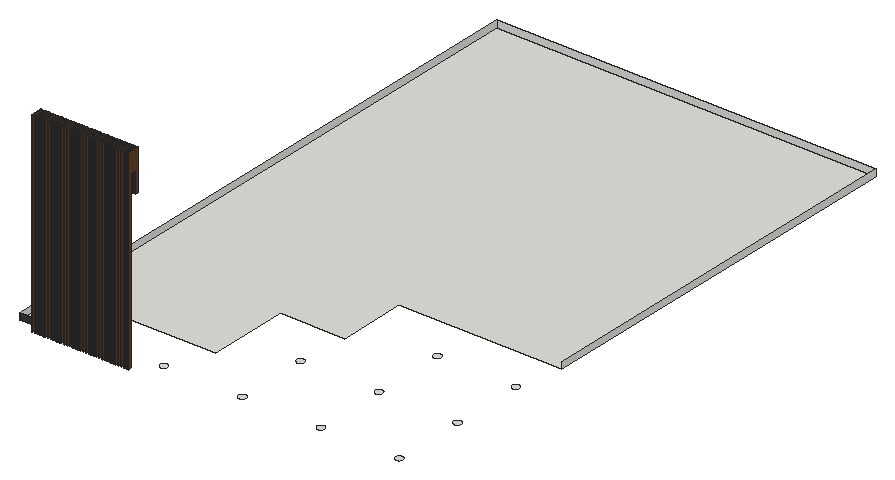
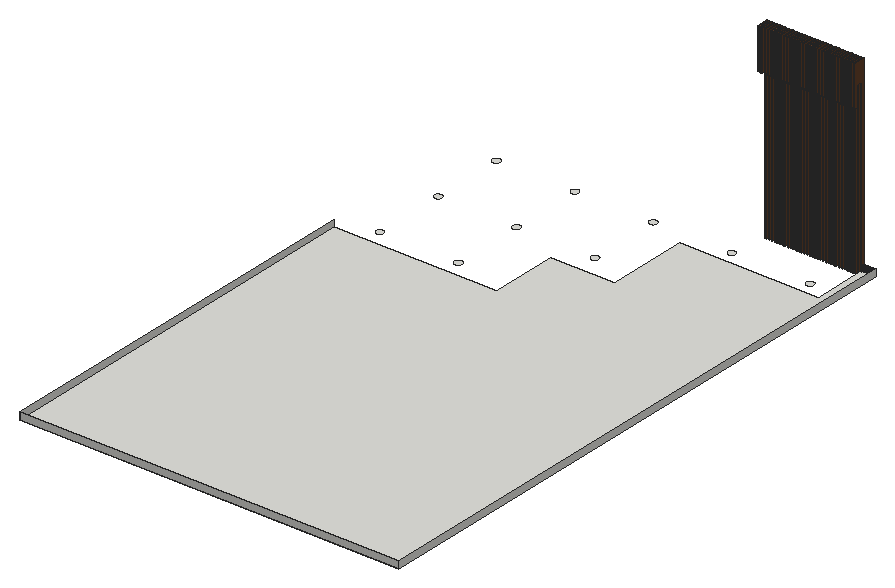
# SketchUp Ruby script. Lengths in inches.
U = 1.inch
M = Sketchup.active_model
def pt(a) = Geom::Point3d.new(a.map { |v| v * U })
def face(e, loops, mat)
  f = e.add_face(loops[0].map { |a| pt(a) })
  loops[1..].each { |l| e.add_face(l.map { |a| pt(a) }).erase! }
  f.material = f.back_material = mat if mat
  f
end
# faces: each face lists its corners as indices into pts; further lists are holes
def faces(e, pts, list, mat = nil) = list.each { |f| face(e, (f[0].is_a?(Array) ? f : [f]).map { |l| l.map { |i| pts[i] } }, mat) }
# xy, xz, yz: faces in a plane at the given z, y or x. An outline is a flat list of corners, or four numbers for a rectangle; further outlines are holes
def ring(l) = l.size == 4 ? [[l[0], l[1]], [l[2], l[1]], [l[2], l[3]], [l[0], l[3]]] : l.each_slice(2).to_a
def flat(e, list, mat, &to3) = list.each { |f| face(e, (f[0].is_a?(Array) ? f : [f]).map { |l| ring(l).map { |u, v| to3.(u, v) } }, mat) }
def xy(e, z, list, mat = nil) = flat(e, list, mat) { |x, y| [x, y, z] }
def xz(e, y, list, mat = nil) = flat(e, list, mat) { |x, z| [x, y, z] }
def yz(e, x, list, mat = nil) = flat(e, list, mat) { |y, z| [x, y, z] }
def lines(e, pts, list) = list.each { |a, b| e.add_line(pt(pts[a]), pt(pts[b])) }
# prism: a flat outline (further loops are holes) pulled along v
def prism(e, loops, v, mat = nil)
  f = face(e, loops, mat); d = Geom::Vector3d.new(v.map { |x| x * U })
  f.pushpull(f.normal.samedirection?(d) ? d.length : -d.length)
end
def box(e, o, s, mat = nil) = prism(e, [[o, [o[0] + s[0], o[1], o[2]], [o[0] + s[0], o[1] + s[1], o[2]], [o[0], o[1] + s[1], o[2]]]], [0, 0, s[2]], mat)
def at(x, y, z, deg = 0) = Geom::Transformation.translation(pt([x, y, z])) * Geom::Transformation.rotation(ORIGIN, Z_AXIS, deg.degrees)
def axes(o, x, y, z) = Geom::Transformation.new([*x, 0, *y, 0, *z, 0, *pt(o).to_a, 1])
def part(name) = M.definitions.add(name)
# library, detail: a bought-in or finely detailed component or shape, given as its bounding box
def library(name, o, s) = part(name).tap { |d| box(d.entities, o, s) }
def detail(e, o, s) = box(e.add_group.entities, o, s)
def put(e, d, t, mat = nil) = e.add_instance(d, t).tap { |i| i.material = mat if mat }
def group(e, t, mat = nil) = e.add_group.tap { |g| g.transformation = t; g.material = mat if mat }.entities
root = M.entities
M.materials.add("1432 AP 8245 TAR ROAD").color = [57, 57, 60]
M.materials.add("[Wood Veneer 01]").color = [99, 65, 42]
c1 = part("2")
prism(c1.entities,[[[0,1.5,0],[0,-0.5,0],[0,-0.5,172],[0,9.5,172],[0,9.5,136],[0,7.5,136],[0,7.5,154],[0,1.5,154]]],[1.5,0,0])
xy(root,111,[[50.84,185,50.76,185.01,50.6875,185.02,50.61,185.03,50.45,185.05,50.375,185.07,50.3,185.08,50.22,185.1,50.15,185.125,50.07,185.15,50,185.17,49.92,185.2,49.71,185.29,49.64,185.33,49.57,185.36,49.43,185.44,49.37,185.48,49.3,185.53,49.24,185.57,49.17,185.62,48.93,185.82,48.88,185.88,48.82,185.93,48.62,186.17,48.57,186.24,48.53,186.3,48.48,186.37,48.44,186.43,48.36,186.57,48.33,186.64,48.29,186.71,48.2,186.92,48.17,187,48.15,187.07,48.125,187.15,48.1,187.22,48.08,187.3,48.07,187.375,48.05,187.45,48.03,187.61,48.02,187.6875,48.01,187.76,48,187.84,48,188.16,48.01,188.24,48.02,188.3125,48.03,188.39,48.05,188.55,48.07,188.625,48.08,188.7,48.1,188.78,48.125,188.85,48.15,188.93,48.17,189,48.2,189.08,48.29,189.29,48.33,189.36,48.36,189.43,48.44,189.57,48.48,189.63,48.53,189.7,48.57,189.76,48.62,189.83,48.82,190.07,48.88,190.12,48.93,190.18,49.17,190.38,49.24,190.43,49.3,190.47,49.37,190.52,49.43,190.56,49.57,190.64,49.64,190.67,49.71,190.71,49.92,190.8,50,190.83,50.07,190.85,50.15,190.875,50.22,190.9,50.3,190.92,50.375,190.93,50.45,190.95,50.61,190.97,50.6875,190.98,50.76,190.99,50.84,191,51.16,191,51.24,190.99,51.3125,190.98,51.39,190.97,51.55,190.95,51.625,190.93,51.7,190.92,51.78,190.9,51.85,190.875,51.93,190.85,52,190.83,52.08,190.8,52.29,190.71,52.36,190.67,52.43,190.64,52.57,190.56,52.63,190.52,52.7,190.47,52.76,190.43,52.83,190.38,53.07,190.18,53.12,190.12,53.18,190.07,53.38,189.83,53.43,189.76,53.47,189.7,53.52,189.63,53.56,189.57,53.64,189.43,53.67,189.36,53.71,189.29,53.8,189.08,53.83,189,53.85,188.93,53.875,188.85,53.9,188.78,53.92,188.7,53.93,188.625,53.95,188.55,53.97,188.39,53.98,188.3125,53.99,188.24,54,188.16,54,187.84,53.99,187.76,53.98,187.6875,53.97,187.61,53.95,187.45,53.93,187.375,53.92,187.3,53.9,187.22,53.875,187.15,53.85,187.07,53.83,187,53.8,186.92,53.71,186.71,53.67,186.64,53.64,186.57,53.56,186.43,53.52,186.37,53.47,186.3,53.43,186.24,53.38,186.17,53.18,185.93,53.12,185.88,53.07,185.82,52.83,185.62,52.76,185.57,52.7,185.53,52.63,185.48,52.57,185.44,52.43,185.36,52.36,185.33,52.29,185.29,52.08,185.2,52,185.17,51.93,185.15,51.85,185.125,51.78,185.1,51.7,185.08,51.625,185.07,51.55,185.05,51.39,185.03,51.3125,185.02,51.24,185.01,51.16,185],[120.34,185,120.26,185.01,120.1875,185.02,120.11,185.03,119.95,185.05,119.875,185.07,119.8,185.08,119.72,185.1,119.65,185.125,119.57,185.15,119.5,185.17,119.42,185.2,119.21,185.29,119.14,185.33,119.07,185.36,118.93,185.44,118.87,185.48,118.8,185.53,118.74,185.57,118.67,185.62,118.43,185.82,118.38,185.88,118.32,185.93,118.12,186.17,118.07,186.24,118.03,186.3,117.98,186.37,117.94,186.43,117.86,186.57,117.83,186.64,117.79,186.71,117.7,186.92,117.67,187,117.65,187.07,117.625,187.15,117.6,187.22,117.58,187.3,117.57,187.375,117.55,187.45,117.53,187.61,117.52,187.6875,117.51,187.76,117.5,187.84,117.5,188.16,117.51,188.24,117.52,188.3125,117.53,188.39,117.55,188.55,117.57,188.625,117.58,188.7,117.6,188.78,117.625,188.85,117.65,188.93,117.67,189,117.7,189.08,117.79,189.29,117.83,189.36,117.86,189.43,117.94,189.57,117.98,189.63,118.03,189.7,118.07,189.76,118.12,189.83,118.32,190.07,118.38,190.12,118.43,190.18,118.67,190.38,118.74,190.43,118.8,190.47,118.87,190.52,118.93,190.56,119.07,190.64,119.14,190.67,119.21,190.71,119.42,190.8,119.5,190.83,119.57,190.85,119.65,190.875,119.72,190.9,119.8,190.92,119.875,190.93,119.95,190.95,120.11,190.97,120.1875,190.98,120.26,190.99,120.34,191,120.66,191,120.74,190.99,120.8125,190.98,120.89,190.97,121.05,190.95,121.125,190.93,121.2,190.92,121.28,190.9,121.35,190.875,121.43,190.85,121.5,190.83,121.58,190.8,121.79,190.71,121.86,190.67,121.93,190.64,122.07,190.56,122.13,190.52,122.2,190.47,122.26,190.43,122.33,190.38,122.57,190.18,122.62,190.12,122.68,190.07,122.88,189.83,122.93,189.76,122.97,189.7,123.02,189.63,123.06,189.57,123.14,189.43,123.17,189.36,123.21,189.29,123.3,189.08,123.33,189,123.35,188.93,123.375,188.85,123.4,188.78,123.42,188.7,123.43,188.625,123.45,188.55,123.47,188.39,123.48,188.3125,123.49,188.24,123.5,188.16,123.5,187.84,123.49,187.76,123.48,187.6875,123.47,187.61,123.45,187.45,123.43,187.375,123.42,187.3,123.4,187.22,123.375,187.15,123.35,187.07,123.33,187,123.3,186.92,123.21,186.71,123.17,186.64,123.14,186.57,123.06,186.43,123.02,186.37,122.97,186.3,122.93,186.24,122.88,186.17,122.68,185.93,122.62,185.88,122.57,185.82,122.33,185.62,122.26,185.57,122.2,185.53,122.13,185.48,122.07,185.44,121.93,185.36,121.86,185.33,121.79,185.29,121.58,185.2,121.5,185.17,121.43,185.15,121.35,185.125,121.28,185.1,121.2,185.08,121.125,185.07,121.05,185.05,120.89,185.03,120.8125,185.02,120.74,185.01,120.66,185],[189.84,185,189.76,185.01,189.6875,185.02,189.61,185.03,189.45,185.05,189.375,185.07,189.3,185.08,189.22,185.1,189.15,185.125,189.07,185.15,189,185.17,188.92,185.2,188.71,185.29,188.64,185.33,188.57,185.36,188.43,185.44,188.37,185.48,188.3,185.53,188.24,185.57,188.17,185.62,187.93,185.82,187.88,185.88,187.82,185.93,187.62,186.17,187.57,186.24,187.53,186.3,187.48,186.37,187.44,186.43,187.36,186.57,187.33,186.64,187.29,186.71,187.2,186.92,187.17,187,187.15,187.07,187.125,187.15,187.1,187.22,187.08,187.3,187.07,187.375,187.05,187.45,187.03,187.61,187.02,187.6875,187.01,187.76,187,187.84,187,188.16,187.01,188.24,187.02,188.3125,187.03,188.39,187.05,188.55,187.07,188.625,187.08,188.7,187.1,188.78,187.125,188.85,187.15,188.93,187.17,189,187.2,189.08,187.29,189.29,187.33,189.36,187.36,189.43,187.44,189.57,187.48,189.63,187.53,189.7,187.57,189.76,187.62,189.83,187.82,190.07,187.88,190.12,187.93,190.18,188.17,190.38,188.24,190.43,188.3,190.47,188.37,190.52,188.43,190.56,188.57,190.64,188.64,190.67,188.71,190.71,188.92,190.8,189,190.83,189.07,190.85,189.15,190.875,189.22,190.9,189.3,190.92,189.375,190.93,189.45,190.95,189.61,190.97,189.6875,190.98,189.76,190.99,189.84,191,190.16,191,190.24,190.99,190.3125,190.98,190.39,190.97,190.55,190.95,190.625,190.93,190.7,190.92,190.78,190.9,190.85,190.875,190.93,190.85,191,190.83,191.08,190.8,191.29,190.71,191.36,190.67,191.43,190.64,191.57,190.56,191.63,190.52,191.7,190.47,191.76,190.43,191.83,190.38,192.07,190.18,192.12,190.12,192.18,190.07,192.38,189.83,192.43,189.76,192.47,189.7,192.52,189.63,192.56,189.57,192.64,189.43,192.67,189.36,192.71,189.29,192.8,189.08,192.83,189,192.85,188.93,192.875,188.85,192.9,188.78,192.92,188.7,192.93,188.625,192.95,188.55,192.97,188.39,192.98,188.3125,192.99,188.24,193,188.16,193,187.84,192.99,187.76,192.98,187.6875,192.97,187.61,192.95,187.45,192.93,187.375,192.92,187.3,192.9,187.22,192.875,187.15,192.85,187.07,192.83,187,192.8,186.92,192.71,186.71,192.67,186.64,192.64,186.57,192.56,186.43,192.52,186.37,192.47,186.3,192.43,186.24,192.38,186.17,192.18,185.93,192.12,185.88,192.07,185.82,191.83,185.62,191.76,185.57,191.7,185.53,191.63,185.48,191.57,185.44,191.43,185.36,191.36,185.33,191.29,185.29,191.08,185.2,191,185.17,190.93,185.15,190.85,185.125,190.78,185.1,190.7,185.08,190.625,185.07,190.55,185.05,190.39,185.03,190.3125,185.02,190.24,185.01,190.16,185],[259.34,185,259.26,185.01,259.1875,185.02,259.11,185.03,258.95,185.05,258.875,185.07,258.8,185.08,258.72,185.1,258.65,185.125,258.57,185.15,258.5,185.17,258.42,185.2,258.21,185.29,258.14,185.33,258.07,185.36,257.93,185.44,257.87,185.48,257.8,185.53,257.74,185.57,257.67,185.62,257.43,185.82,257.38,185.88,257.32,185.93,257.12,186.17,257.07,186.24,257.03,186.3,256.98,186.37,256.94,186.43,256.86,186.57,256.83,186.64,256.79,186.71,256.7,186.92,256.67,187,256.65,187.07,256.625,187.15,256.6,187.22,256.58,187.3,256.57,187.375,256.55,187.45,256.53,187.61,256.52,187.6875,256.51,187.76,256.5,187.84,256.5,188.16,256.51,188.24,256.52,188.3125,256.53,188.39,256.55,188.55,256.57,188.625,256.58,188.7,256.6,188.78,256.625,188.85,256.65,188.93,256.67,189,256.7,189.08,256.79,189.29,256.83,189.36,256.86,189.43,256.94,189.57,256.98,189.63,257.03,189.7,257.07,189.76,257.12,189.83,257.32,190.07,257.38,190.12,257.43,190.18,257.67,190.38,257.74,190.43,257.8,190.47,257.87,190.52,257.93,190.56,258.07,190.64,258.14,190.67,258.21,190.71,258.42,190.8,258.5,190.83,258.57,190.85,258.65,190.875,258.72,190.9,258.8,190.92,258.875,190.93,258.95,190.95,259.11,190.97,259.1875,190.98,259.26,190.99,259.34,191,259.66,191,259.74,190.99,259.8125,190.98,259.89,190.97,260.05,190.95,260.125,190.93,260.2,190.92,260.28,190.9,260.35,190.875,260.43,190.85,260.5,190.83,260.58,190.8,260.79,190.71,260.86,190.67,260.93,190.64,261.07,190.56,261.13,190.52,261.2,190.47,261.26,190.43,261.33,190.38,261.57,190.18,261.62,190.12,261.68,190.07,261.88,189.83,261.93,189.76,261.97,189.7,262.02,189.63,262.06,189.57,262.14,189.43,262.17,189.36,262.21,189.29,262.3,189.08,262.33,189,262.35,188.93,262.375,188.85,262.4,188.78,262.42,188.7,262.43,188.625,262.45,188.55,262.47,188.39,262.48,188.3125,262.49,188.24,262.5,188.16,262.5,187.84,262.49,187.76,262.48,187.6875,262.47,187.61,262.45,187.45,262.43,187.375,262.42,187.3,262.4,187.22,262.375,187.15,262.35,187.07,262.33,187,262.3,186.92,262.21,186.71,262.17,186.64,262.14,186.57,262.06,186.43,262.02,186.37,261.97,186.3,261.93,186.24,261.88,186.17,261.68,185.93,261.62,185.88,261.57,185.82,261.33,185.62,261.26,185.57,261.2,185.53,261.13,185.48,261.07,185.44,260.93,185.36,260.86,185.33,260.79,185.29,260.58,185.2,260.5,185.17,260.43,185.15,260.35,185.125,260.28,185.1,260.2,185.08,260.125,185.07,260.05,185.05,259.89,185.03,259.8125,185.02,259.74,185.01,259.66,185],[328.84,185,328.76,185.01,328.6875,185.02,328.61,185.03,328.45,185.05,328.375,185.07,328.3,185.08,328.22,185.1,328.15,185.125,328.07,185.15,328,185.17,327.92,185.2,327.71,185.29,327.64,185.33,327.57,185.36,327.43,185.44,327.37,185.48,327.3,185.53,327.24,185.57,327.17,185.62,326.93,185.82,326.88,185.88,326.82,185.93,326.62,186.17,326.57,186.24,326.53,186.3,326.48,186.37,326.44,186.43,326.36,186.57,326.33,186.64,326.29,186.71,326.2,186.92,326.17,187,326.15,187.07,326.125,187.15,326.1,187.22,326.08,187.3,326.07,187.375,326.05,187.45,326.03,187.61,326.02,187.6875,326.01,187.76,326,187.84,326,188.16,326.01,188.24,326.02,188.3125,326.03,188.39,326.05,188.55,326.07,188.625,326.08,188.7,326.1,188.78,326.125,188.85,326.15,188.93,326.17,189,326.2,189.08,326.29,189.29,326.33,189.36,326.36,189.43,326.44,189.57,326.48,189.63,326.53,189.7,326.57,189.76,326.62,189.83,326.82,190.07,326.88,190.12,326.93,190.18,327.17,190.38,327.24,190.43,327.3,190.47,327.37,190.52,327.43,190.56,327.57,190.64,327.64,190.67,327.71,190.71,327.92,190.8,328,190.83,328.07,190.85,328.15,190.875,328.22,190.9,328.3,190.92,328.375,190.93,328.45,190.95,328.61,190.97,328.6875,190.98,328.76,190.99,328.84,191,329.16,191,329.24,190.99,329.3125,190.98,329.39,190.97,329.55,190.95,329.625,190.93,329.7,190.92,329.78,190.9,329.85,190.875,329.93,190.85,330,190.83,330.08,190.8,330.29,190.71,330.36,190.67,330.43,190.64,330.57,190.56,330.63,190.52,330.7,190.47,330.76,190.43,330.83,190.38,331.07,190.18,331.12,190.12,331.18,190.07,331.38,189.83,331.43,189.76,331.47,189.7,331.52,189.63,331.56,189.57,331.64,189.43,331.67,189.36,331.71,189.29,331.8,189.08,331.83,189,331.85,188.93,331.875,188.85,331.9,188.78,331.92,188.7,331.93,188.625,331.95,188.55,331.97,188.39,331.98,188.3125,331.99,188.24,332,188.16,332,187.84,331.99,187.76,331.98,187.6875,331.97,187.61,331.95,187.45,331.93,187.375,331.92,187.3,331.9,187.22,331.875,187.15,331.85,187.07,331.83,187,331.8,186.92,331.71,186.71,331.67,186.64,331.64,186.57,331.56,186.43,331.52,186.37,331.47,186.3,331.43,186.24,331.38,186.17,331.18,185.93,331.12,185.88,331.07,185.82,330.83,185.62,330.76,185.57,330.7,185.53,330.63,185.48,330.57,185.44,330.43,185.36,330.36,185.33,330.29,185.29,330.08,185.2,330,185.17,329.93,185.15,329.85,185.125,329.78,185.1,329.7,185.08,329.625,185.07,329.55,185.05,329.39,185.03,329.3125,185.02,329.24,185.01,329.16,185],
  [189.84,249.5,189.76,249.51,189.6875,249.52,189.61,249.53,189.45,249.55,189.375,249.57,189.3,249.58,189.22,249.6,189.15,249.625,189.07,249.65,189,249.67,188.92,249.7,188.71,249.79,188.64,249.83,188.57,249.86,188.43,249.94,188.37,249.98,188.3,250.03,188.24,250.07,188.17,250.12,187.93,250.32,187.88,250.38,187.82,250.43,187.62,250.67,187.57,250.74,187.53,250.8,187.48,250.87,187.44,250.93,187.36,251.07,187.33,251.14,187.29,251.21,187.2,251.42,187.17,251.5,187.15,251.57,187.125,251.65,187.1,251.72,187.08,251.8,187.07,251.875,187.05,251.95,187.03,252.11,187.02,252.1875,187.01,252.26,187,252.34,187,252.66,187.01,252.74,187.02,252.8125,187.03,252.89,187.05,253.05,187.07,253.125,187.08,253.2,187.1,253.28,187.125,253.35,187.15,253.43,187.17,253.5,187.2,253.58,187.29,253.79,187.33,253.86,187.36,253.93,187.44,254.07,187.48,254.13,187.53,254.2,187.57,254.26,187.62,254.33,187.82,254.57,187.88,254.62,187.93,254.68,188.17,254.88,188.24,254.93,188.3,254.97,188.37,255.02,188.43,255.06,188.57,255.14,188.64,255.17,188.71,255.21,188.92,255.3,189,255.33,189.07,255.35,189.15,255.375,189.22,255.4,189.3,255.42,189.375,255.43,189.45,255.45,189.61,255.47,189.6875,255.48,189.76,255.49,189.84,255.5,190.16,255.5,190.24,255.49,190.3125,255.48,190.39,255.47,190.55,255.45,190.625,255.43,190.7,255.42,190.78,255.4,190.85,255.375,190.93,255.35,191,255.33,191.08,255.3,191.29,255.21,191.36,255.17,191.43,255.14,191.57,255.06,191.63,255.02,191.7,254.97,191.76,254.93,191.83,254.88,192.07,254.68,192.12,254.62,192.18,254.57,192.38,254.33,192.43,254.26,192.47,254.2,192.52,254.13,192.56,254.07,192.64,253.93,192.67,253.86,192.71,253.79,192.8,253.58,192.83,253.5,192.85,253.43,192.875,253.35,192.9,253.28,192.92,253.2,192.93,253.125,192.95,253.05,192.97,252.89,192.98,252.8125,192.99,252.74,193,252.66,193,252.34,192.99,252.26,192.98,252.1875,192.97,252.11,192.95,251.95,192.93,251.875,192.92,251.8,192.9,251.72,192.875,251.65,192.85,251.57,192.83,251.5,192.8,251.42,192.71,251.21,192.67,251.14,192.64,251.07,192.56,250.93,192.52,250.87,192.47,250.8,192.43,250.74,192.38,250.67,192.18,250.43,192.12,250.38,192.07,250.32,191.83,250.12,191.76,250.07,191.7,250.03,191.63,249.98,191.57,249.94,191.43,249.86,191.36,249.83,191.29,249.79,191.08,249.7,191,249.67,190.93,249.65,190.85,249.625,190.78,249.6,190.7,249.58,190.625,249.57,190.55,249.55,190.39,249.53,190.3125,249.52,190.24,249.51,190.16,249.5],[259.34,249.5,259.26,249.51,259.1875,249.52,259.11,249.53,258.95,249.55,258.875,249.57,258.8,249.58,258.72,249.6,258.65,249.625,258.57,249.65,258.5,249.67,258.42,249.7,258.21,249.79,258.14,249.83,258.07,249.86,257.93,249.94,257.87,249.98,257.8,250.03,257.74,250.07,257.67,250.12,257.43,250.32,257.38,250.38,257.32,250.43,257.12,250.67,257.07,250.74,257.03,250.8,256.98,250.87,256.94,250.93,256.86,251.07,256.83,251.14,256.79,251.21,256.7,251.42,256.67,251.5,256.65,251.57,256.625,251.65,256.6,251.72,256.58,251.8,256.57,251.875,256.55,251.95,256.53,252.11,256.52,252.1875,256.51,252.26,256.5,252.34,256.5,252.66,256.51,252.74,256.52,252.8125,256.53,252.89,256.55,253.05,256.57,253.125,256.58,253.2,256.6,253.28,256.625,253.35,256.65,253.43,256.67,253.5,256.7,253.58,256.79,253.79,256.83,253.86,256.86,253.93,256.94,254.07,256.98,254.13,257.03,254.2,257.07,254.26,257.12,254.33,257.32,254.57,257.38,254.62,257.43,254.68,257.67,254.88,257.74,254.93,257.8,254.97,257.87,255.02,257.93,255.06,258.07,255.14,258.14,255.17,258.21,255.21,258.42,255.3,258.5,255.33,258.57,255.35,258.65,255.375,258.72,255.4,258.8,255.42,258.875,255.43,258.95,255.45,259.11,255.47,259.1875,255.48,259.26,255.49,259.34,255.5,259.66,255.5,259.74,255.49,259.8125,255.48,259.89,255.47,260.05,255.45,260.125,255.43,260.2,255.42,260.28,255.4,260.35,255.375,260.43,255.35,260.5,255.33,260.58,255.3,260.79,255.21,260.86,255.17,260.93,255.14,261.07,255.06,261.13,255.02,261.2,254.97,261.26,254.93,261.33,254.88,261.57,254.68,261.62,254.62,261.68,254.57,261.88,254.33,261.93,254.26,261.97,254.2,262.02,254.13,262.06,254.07,262.14,253.93,262.17,253.86,262.21,253.79,262.3,253.58,262.33,253.5,262.35,253.43,262.375,253.35,262.4,253.28,262.42,253.2,262.43,253.125,262.45,253.05,262.47,252.89,262.48,252.8125,262.49,252.74,262.5,252.66,262.5,252.34,262.49,252.26,262.48,252.1875,262.47,252.11,262.45,251.95,262.43,251.875,262.42,251.8,262.4,251.72,262.375,251.65,262.35,251.57,262.33,251.5,262.3,251.42,262.21,251.21,262.17,251.14,262.14,251.07,262.06,250.93,262.02,250.87,261.97,250.8,261.93,250.74,261.88,250.67,261.68,250.43,261.62,250.38,261.57,250.32,261.33,250.12,261.26,250.07,261.2,250.03,261.13,249.98,261.07,249.94,260.93,249.86,260.86,249.83,260.79,249.79,260.58,249.7,260.5,249.67,260.43,249.65,260.35,249.625,260.28,249.6,260.2,249.58,260.125,249.57,260.05,249.55,259.89,249.53,259.8125,249.52,259.74,249.51,259.66,249.5],[328.84,249.5,328.76,249.51,328.6875,249.52,328.61,249.53,328.45,249.55,328.375,249.57,328.3,249.58,328.22,249.6,328.15,249.625,328.07,249.65,328,249.67,327.92,249.7,327.71,249.79,327.64,249.83,327.57,249.86,327.43,249.94,327.37,249.98,327.3,250.03,327.24,250.07,327.17,250.12,326.93,250.32,326.88,250.38,326.82,250.43,326.62,250.67,326.57,250.74,326.53,250.8,326.48,250.87,326.44,250.93,326.36,251.07,326.33,251.14,326.29,251.21,326.2,251.42,326.17,251.5,326.15,251.57,326.125,251.65,326.1,251.72,326.08,251.8,326.07,251.875,326.05,251.95,326.03,252.11,326.02,252.1875,326.01,252.26,326,252.34,326,252.66,326.01,252.74,326.02,252.8125,326.03,252.89,326.05,253.05,326.07,253.125,326.08,253.2,326.1,253.28,326.125,253.35,326.15,253.43,326.17,253.5,326.2,253.58,326.29,253.79,326.33,253.86,326.36,253.93,326.44,254.07,326.48,254.13,326.53,254.2,326.57,254.26,326.62,254.33,326.82,254.57,326.88,254.62,326.93,254.68,327.17,254.88,327.24,254.93,327.3,254.97,327.37,255.02,327.43,255.06,327.57,255.14,327.64,255.17,327.71,255.21,327.92,255.3,328,255.33,328.07,255.35,328.15,255.375,328.22,255.4,328.3,255.42,328.375,255.43,328.45,255.45,328.61,255.47,328.6875,255.48,328.76,255.49,328.84,255.5,329.16,255.5,329.24,255.49,329.3125,255.48,329.39,255.47,329.55,255.45,329.625,255.43,329.7,255.42,329.78,255.4,329.85,255.375,329.93,255.35,330,255.33,330.08,255.3,330.29,255.21,330.36,255.17,330.43,255.14,330.57,255.06,330.63,255.02,330.7,254.97,330.76,254.93,330.83,254.88,331.07,254.68,331.12,254.62,331.18,254.57,331.38,254.33,331.43,254.26,331.47,254.2,331.52,254.13,331.56,254.07,331.64,253.93,331.67,253.86,331.71,253.79,331.8,253.58,331.83,253.5,331.85,253.43,331.875,253.35,331.9,253.28,331.92,253.2,331.93,253.125,331.95,253.05,331.97,252.89,331.98,252.8125,331.99,252.74,332,252.66,332,252.34,331.99,252.26,331.98,252.1875,331.97,252.11,331.95,251.95,331.93,251.875,331.92,251.8,331.9,251.72,331.875,251.65,331.85,251.57,331.83,251.5,331.8,251.42,331.71,251.21,331.67,251.14,331.64,251.07,331.56,250.93,331.52,250.87,331.47,250.8,331.43,250.74,331.38,250.67,331.18,250.43,331.12,250.38,331.07,250.32,330.83,250.12,330.76,250.07,330.7,250.03,330.63,249.98,330.57,249.94,330.43,249.86,330.36,249.83,330.29,249.79,330.08,249.7,330,249.67,329.93,249.65,329.85,249.625,329.78,249.6,329.7,249.58,329.625,249.57,329.55,249.55,329.39,249.53,329.3125,249.52,329.24,249.51,329.16,249.5],[259.34,314,259.26,314.01,259.1875,314.02,259.11,314.03,258.95,314.05,258.875,314.07,258.8,314.08,258.72,314.1,258.65,314.125,258.57,314.15,258.5,314.17,258.42,314.2,258.21,314.29,258.14,314.33,258.07,314.36,257.93,314.44,257.87,314.48,257.8,314.53,257.74,314.57,257.67,314.62,257.43,314.82,257.38,314.88,257.32,314.93,257.12,315.17,257.07,315.24,257.03,315.3,256.98,315.37,256.94,315.43,256.86,315.57,256.83,315.64,256.79,315.71,256.7,315.92,256.67,316,256.65,316.07,256.625,316.15,256.6,316.22,256.58,316.3,256.57,316.375,256.55,316.45,256.53,316.61,256.52,316.6875,256.51,316.76,256.5,316.84,256.5,317.16,256.51,317.24,256.52,317.3125,256.53,317.39,256.55,317.55,256.57,317.625,256.58,317.7,256.6,317.78,256.625,317.85,256.65,317.93,256.67,318,256.7,318.08,256.79,318.29,256.83,318.36,256.86,318.43,256.94,318.57,256.98,318.63,257.03,318.7,257.07,318.76,257.12,318.83,257.32,319.07,257.38,319.12,257.43,319.18,257.67,319.38,257.74,319.43,257.8,319.47,257.87,319.52,257.93,319.56,258.07,319.64,258.14,319.67,258.21,319.71,258.42,319.8,258.5,319.83,258.57,319.85,258.65,319.875,258.72,319.9,258.8,319.92,258.875,319.93,258.95,319.95,259.11,319.97,259.1875,319.98,259.26,319.99,259.34,320,259.66,320,259.74,319.99,259.8125,319.98,259.89,319.97,260.05,319.95,260.125,319.93,260.2,319.92,260.28,319.9,260.35,319.875,260.43,319.85,260.5,319.83,260.58,319.8,260.79,319.71,260.86,319.67,260.93,319.64,261.07,319.56,261.13,319.52,261.2,319.47,261.26,319.43,261.33,319.38,261.57,319.18,261.62,319.12,261.68,319.07,261.88,318.83,261.93,318.76,261.97,318.7,262.02,318.63,262.06,318.57,262.14,318.43,262.17,318.36,262.21,318.29,262.3,318.08,262.33,318,262.35,317.93,262.375,317.85,262.4,317.78,262.42,317.7,262.43,317.625,262.45,317.55,262.47,317.39,262.48,317.3125,262.49,317.24,262.5,317.16,262.5,316.84,262.49,316.76,262.48,316.6875,262.47,316.61,262.45,316.45,262.43,316.375,262.42,316.3,262.4,316.22,262.375,316.15,262.35,316.07,262.33,316,262.3,315.92,262.21,315.71,262.17,315.64,262.14,315.57,262.06,315.43,262.02,315.37,261.97,315.3,261.93,315.24,261.88,315.17,261.68,314.93,261.62,314.88,261.57,314.82,261.33,314.62,261.26,314.57,261.2,314.53,261.13,314.48,261.07,314.44,260.93,314.36,260.86,314.33,260.79,314.29,260.58,314.2,260.5,314.17,260.43,314.15,260.35,314.125,260.28,314.1,260.2,314.08,260.125,314.07,260.05,314.05,259.89,314.03,259.8125,314.02,259.74,314.01,259.66,314],[328.84,314,328.76,314.01,328.6875,314.02,328.61,314.03,328.45,314.05,328.375,314.07,328.3,314.08,328.22,314.1,328.15,314.125,328.07,314.15,328,314.17,327.92,314.2,327.71,314.29,327.64,314.33,327.57,314.36,327.43,314.44,327.37,314.48,327.3,314.53,327.24,314.57,327.17,314.62,326.93,314.82,326.88,314.88,326.82,314.93,326.62,315.17,326.57,315.24,326.53,315.3,326.48,315.37,326.44,315.43,326.36,315.57,326.33,315.64,326.29,315.71,326.2,315.92,326.17,316,326.15,316.07,326.125,316.15,326.1,316.22,326.08,316.3,326.07,316.375,326.05,316.45,326.03,316.61,326.02,316.6875,326.01,316.76,326,316.84,326,317.16,326.01,317.24,326.02,317.3125,326.03,317.39,326.05,317.55,326.07,317.625,326.08,317.7,326.1,317.78,326.125,317.85,326.15,317.93,326.17,318,326.2,318.08,326.29,318.29,326.33,318.36,326.36,318.43,326.44,318.57,326.48,318.63,326.53,318.7,326.57,318.76,326.62,318.83,326.82,319.07,326.88,319.12,326.93,319.18,327.17,319.38,327.24,319.43,327.3,319.47,327.37,319.52,327.43,319.56,327.57,319.64,327.64,319.67,327.71,319.71,327.92,319.8,328,319.83,328.07,319.85,328.15,319.875,328.22,319.9,328.3,319.92,328.375,319.93,328.45,319.95,328.61,319.97,328.6875,319.98,328.76,319.99,328.84,320,329.16,320,329.24,319.99,329.3125,319.98,329.39,319.97,329.55,319.95,329.625,319.93,329.7,319.92,329.78,319.9,329.85,319.875,329.93,319.85,330,319.83,330.08,319.8,330.29,319.71,330.36,319.67,330.43,319.64,330.57,319.56,330.63,319.52,330.7,319.47,330.76,319.43,330.83,319.38,331.07,319.18,331.12,319.12,331.18,319.07,331.38,318.83,331.43,318.76,331.47,318.7,331.52,318.63,331.56,318.57,331.64,318.43,331.67,318.36,331.71,318.29,331.8,318.08,331.83,318,331.85,317.93,331.875,317.85,331.9,317.78,331.92,317.7,331.93,317.625,331.95,317.55,331.97,317.39,331.98,317.3125,331.99,317.24,332,317.16,332,316.84,331.99,316.76,331.98,316.6875,331.97,316.61,331.95,316.45,331.93,316.375,331.92,316.3,331.9,316.22,331.875,316.15,331.85,316.07,331.83,316,331.8,315.92,331.71,315.71,331.67,315.64,331.64,315.57,331.56,315.43,331.52,315.37,331.47,315.3,331.43,315.24,331.38,315.17,331.18,314.93,331.12,314.88,331.07,314.82,330.83,314.62,330.76,314.57,330.7,314.53,330.63,314.48,330.57,314.44,330.43,314.36,330.36,314.33,330.29,314.29,330.08,314.2,330,314.17,329.93,314.15,329.85,314.125,329.78,314.1,329.7,314.08,329.625,314.07,329.55,314.05,329.39,314.03,329.3125,314.02,329.24,314.01,329.16,314]])
xy(root,120,[[12,164,12,692,348,692,348,344,204,344,204,284,147,284,147,212,24,212,24,164]])
xz(root,164,[[12,120,24,126]],"1432 AP 8245 TAR ROAD")
xz(root,692,[[12,120,348,126]])
yz(root,12,[[164,120,692,126]])
yz(root,348,[[344,120,692,126]])
g1 = group(root,at(24,162.5,116),"[Wood Veneer 01]")
put(g1,c1,at(0,0,0))
put(g1,c1,at(2.82,0,0))
put(g1,c1,at(5.63,0,0))
put(g1,c1,at(8.45,0,0))
put(g1,c1,at(11.27,0,0))
put(g1,c1,at(14.08,0,0))
put(g1,c1,at(16.9,0,0))
put(g1,c1,at(19.72,0,0))
put(g1,c1,at(22.53,0,0))
put(g1,c1,at(25.35,0,0))
put(g1,c1,at(28.17,0,0))
put(g1,c1,at(30.98,0,0))
put(g1,c1,at(33.8,0,0))
put(g1,c1,at(36.62,0,0))
put(g1,c1,at(39.43,0,0))
put(g1,c1,at(42.25,0,0))
put(g1,c1,at(45.07,0,0))
put(g1,c1,at(47.88,0,0))
put(g1,c1,at(50.7,0,0))
put(g1,c1,at(53.52,0,0))
put(g1,c1,at(56.33,0,0))
put(g1,c1,at(59.15,0,0))
put(g1,c1,at(61.97,0,0))
put(g1,c1,at(64.78,0,0))
put(g1,c1,at(67.6,0,0))
put(g1,c1,at(70.42,0,0))
put(g1,c1,at(73.23,0,0))
put(g1,c1,at(76.05,0,0))
put(g1,c1,at(78.87,0,0))
put(g1,c1,at(81.68,0,0))
put(g1,c1,at(84.5,0,0))
